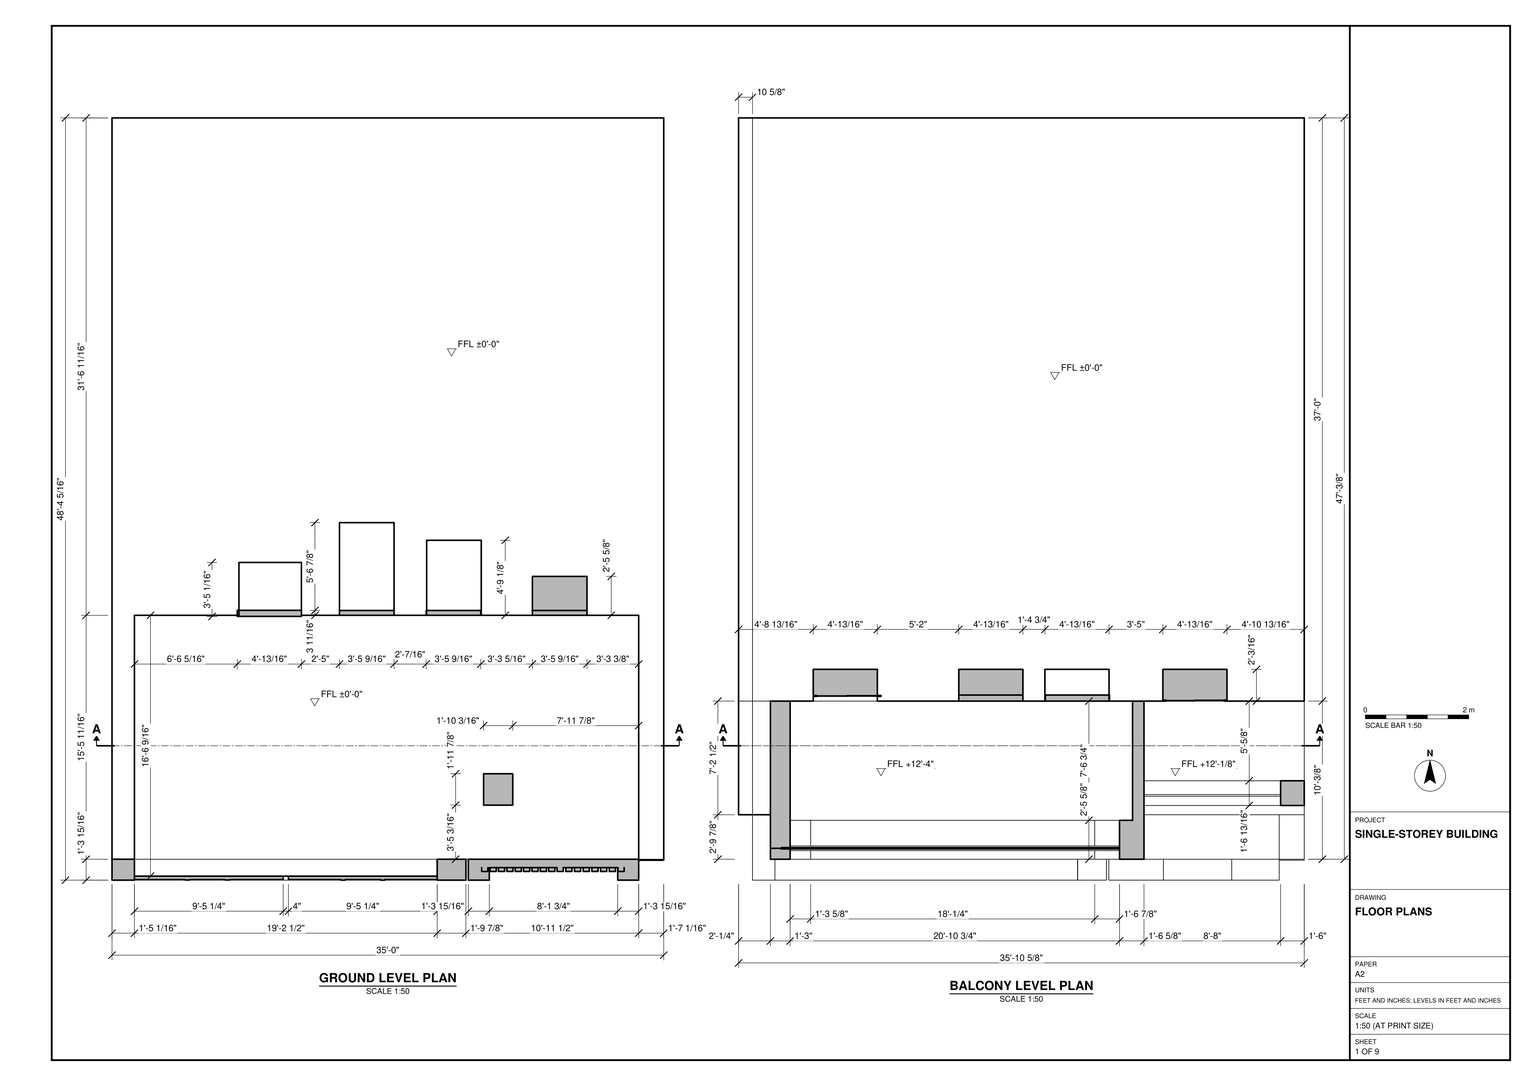
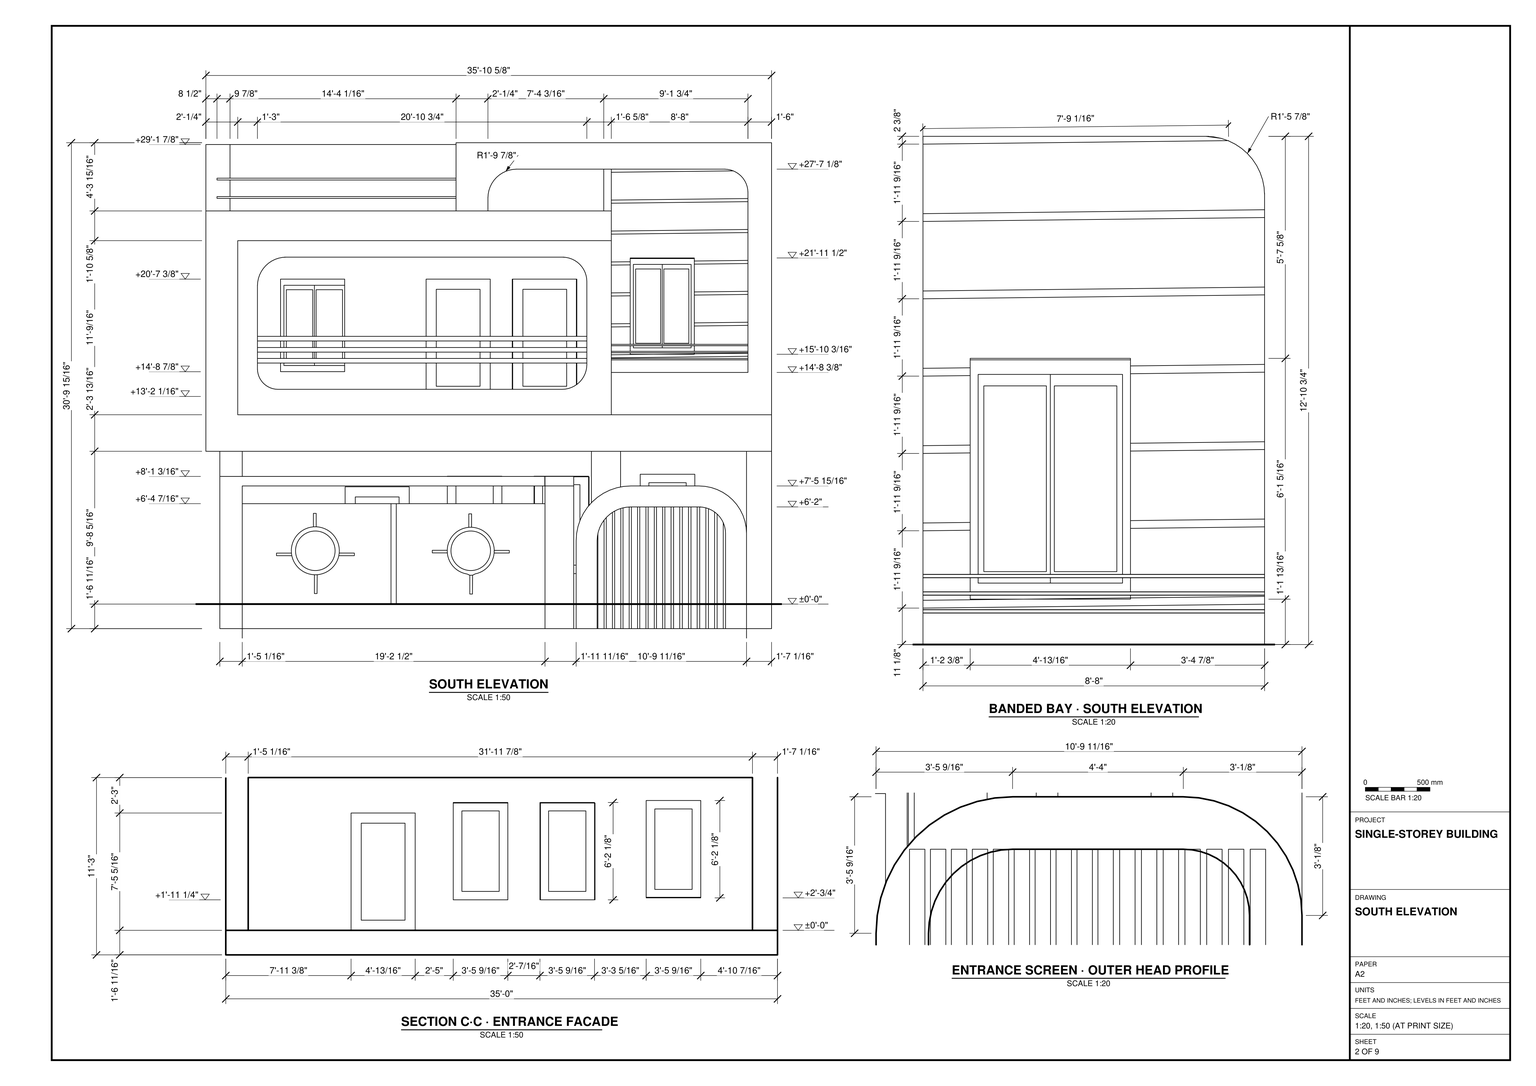
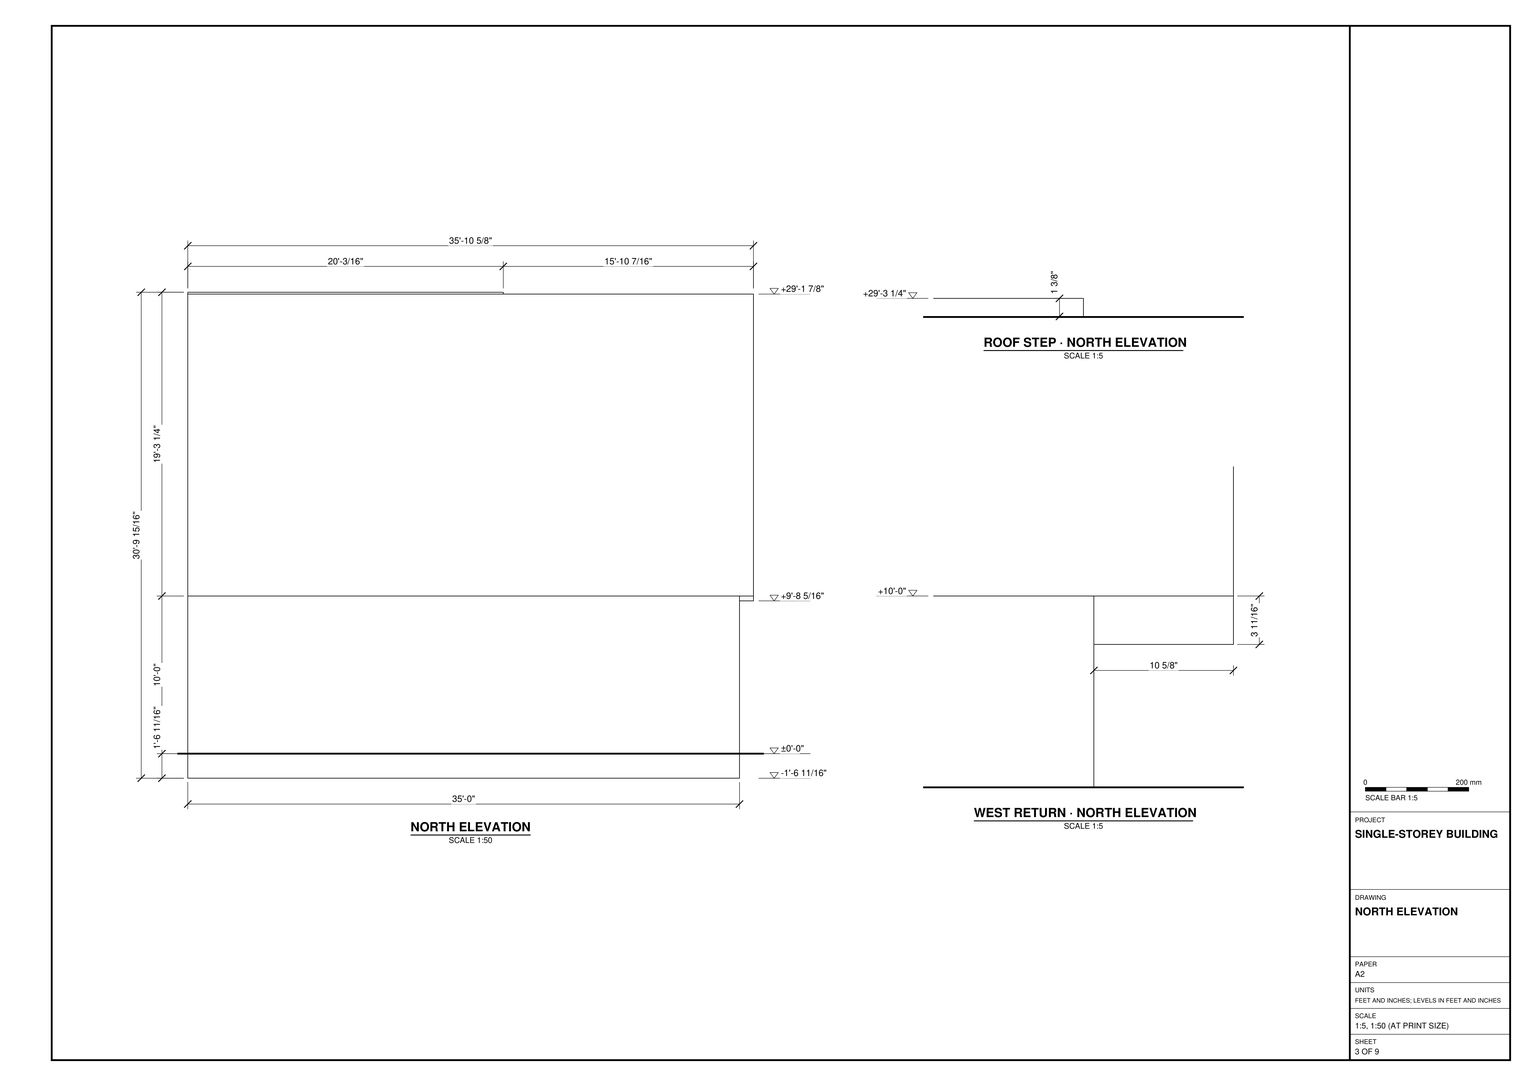
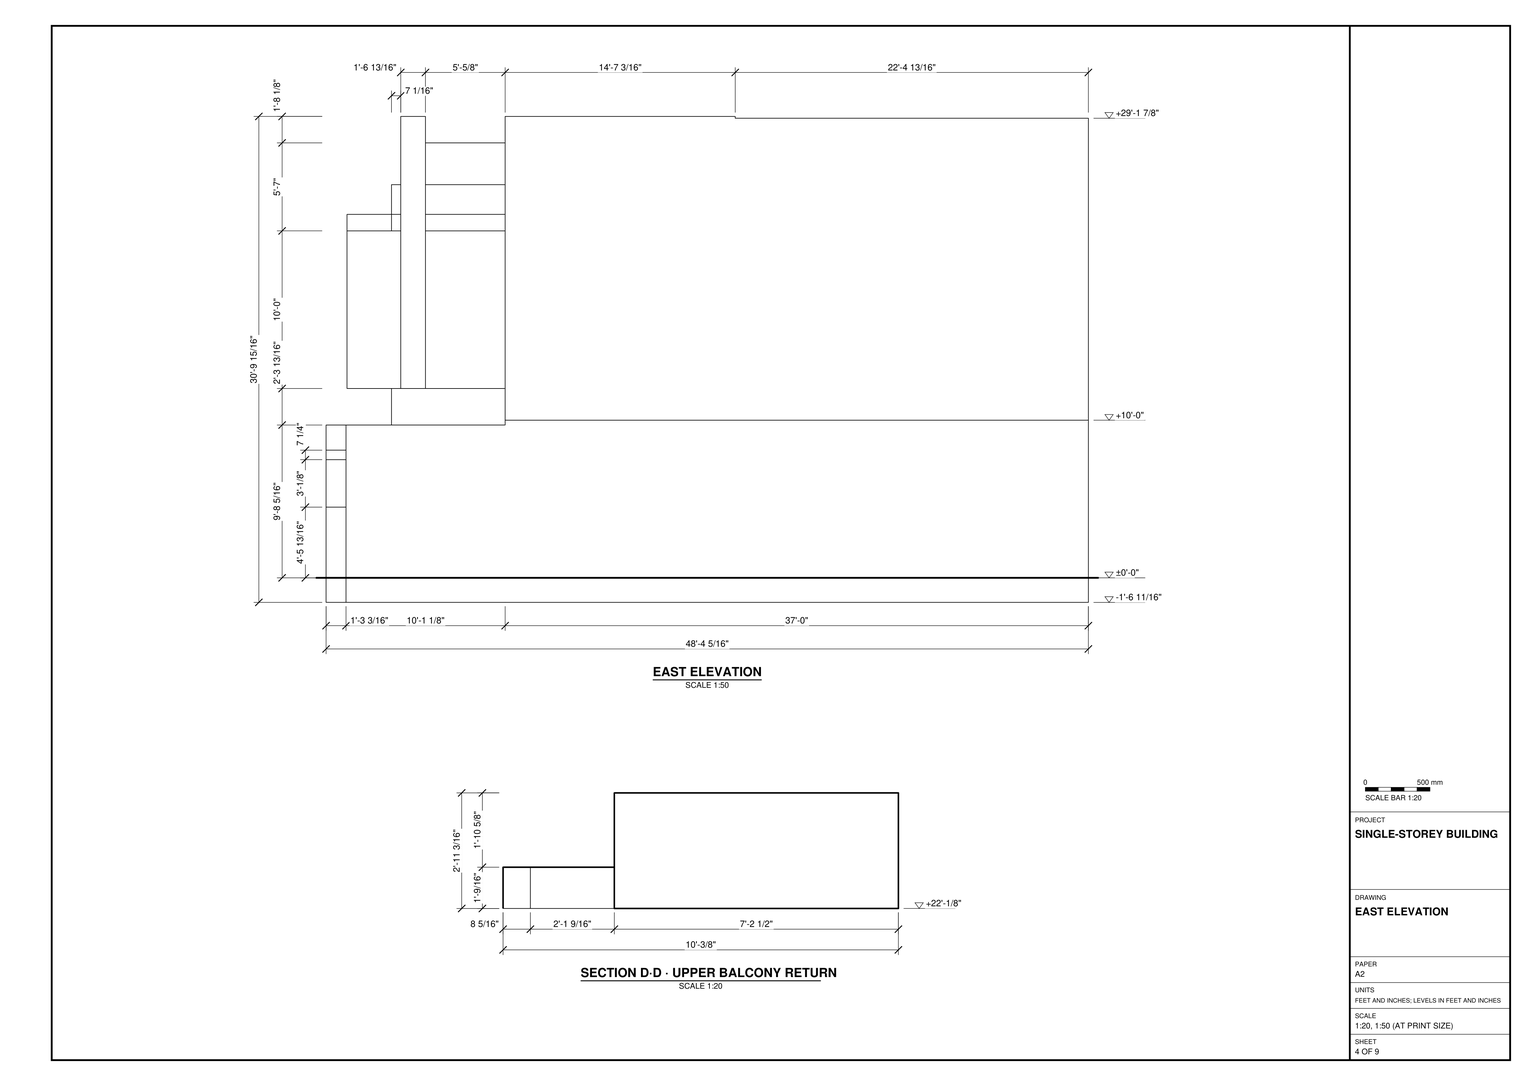
Build the house in SketchUp using the plans, elevations, sections and details in task_files/diagram_01.pdf. Work in feet and inches. Set the ground finished floor at ±0'-0". The overall model dimensions are 35'-10 5/8" wide along X, 48'-4 5/16" deep along Y and 30'-9 15/16" high along Z.

Model the base below the ground floor, the walls at their drawn thicknesses, the floor and balcony slabs, and the roof with its shallow step. At the south entrance, set the wall with the door and windows back from the gate line. Place the broad paired gate on the left and the narrower slatted screen on the right, following the curved head profile in the detail. Above the gate, form the balcony surround with rounded inner corners. Set the openings behind the horizontal guardrails. Model the adjoining banded bay with its paired window and rounded outer corner. Use the north elevation to set out the west return.

Keep walls, slabs, roof and each furniture or joinery piece shown in separate groups or components. Use components for repeated parts such as screen slats. Any decor or loose items shown may be suitable library components. Save one SketchUp model as output_files/single_storey_house_with_a_framed_south_balcony.skp.

# SketchUp Ruby script. Lengths in inches.
U = 1.inch
M = Sketchup.active_model
def pt(a) = Geom::Point3d.new(a.map { |v| v * U })
def face(e, loops, mat)
  f = e.add_face(loops[0].map { |a| pt(a) })
  loops[1..].each { |l| e.add_face(l.map { |a| pt(a) }).erase! }
  f.material = f.back_material = mat if mat
  f
end
# faces: each face lists its corners as indices into pts; further lists are holes
def faces(e, pts, list, mat = nil) = list.each { |f| face(e, (f[0].is_a?(Array) ? f : [f]).map { |l| l.map { |i| pts[i] } }, mat) }
# xy, xz, yz: faces in a plane at the given z, y or x. An outline is a flat list of corners, or four numbers for a rectangle; further outlines are holes
def ring(l) = l.size == 4 ? [[l[0], l[1]], [l[2], l[1]], [l[2], l[3]], [l[0], l[3]]] : l.each_slice(2).to_a
def flat(e, list, mat, &to3) = list.each { |f| face(e, (f[0].is_a?(Array) ? f : [f]).map { |l| ring(l).map { |u, v| to3.(u, v) } }, mat) }
def xy(e, z, list, mat = nil) = flat(e, list, mat) { |x, y| [x, y, z] }
def xz(e, y, list, mat = nil) = flat(e, list, mat) { |x, z| [x, y, z] }
def yz(e, x, list, mat = nil) = flat(e, list, mat) { |y, z| [x, y, z] }
def lines(e, pts, list) = list.each { |a, b| e.add_line(pt(pts[a]), pt(pts[b])) }
# prism: a flat outline (further loops are holes) pulled along v
def prism(e, loops, v, mat = nil)
  f = face(e, loops, mat); d = Geom::Vector3d.new(v.map { |x| x * U })
  f.pushpull(f.normal.samedirection?(d) ? d.length : -d.length)
end
def box(e, o, s, mat = nil) = prism(e, [[o, [o[0] + s[0], o[1], o[2]], [o[0] + s[0], o[1] + s[1], o[2]], [o[0], o[1] + s[1], o[2]]]], [0, 0, s[2]], mat)
def at(x, y, z, deg = 0) = Geom::Transformation.translation(pt([x, y, z])) * Geom::Transformation.rotation(ORIGIN, Z_AXIS, deg.degrees)
def axes(o, x, y, z) = Geom::Transformation.new([*x, 0, *y, 0, *z, 0, *pt(o).to_a, 1])
def part(name) = M.definitions.add(name)
# library, detail: a bought-in or finely detailed component or shape, given as its bounding box
def library(name, o, s) = part(name).tap { |d| box(d.entities, o, s) }
def detail(e, o, s) = box(e.add_group.entities, o, s)
def put(e, d, t, mat = nil) = e.add_instance(d, t).tap { |i| i.material = mat if mat }
def group(e, t, mat = nil) = e.add_group.tap { |g| g.transformation = t; g.material = mat if mat }.entities
root = M.entities
M.materials.add("Generic").color = [106, 57, 18]
M.materials.add("Generic\#1").color = [226, 203, 162]
M.materials.add("Generic\#2").color = [238, 245, 255]
M.materials.add("Generic\#3").color = [229, 166, 115]
M.materials.add("Generic\#4").color = [129, 129, 129]
M.materials.add("Generic\#5").color = [200, 187, 187]
M.materials.add("[Color M07]").color = [58, 58, 58]
M.materials.add("[Translucent Glass Gray]").color = [128, 128, 128]
M.materials["[Translucent Glass Gray]"].alpha = 0.5
M.materials.add("[Wood Veneer 01]").color = [120, 70, 37]
c1 = library("Sliding window",[0,0,0],[4.33,55.51,41.34])
c2 = part("Group\#1")
xz(c2.entities,0,[[0,0,4.6875,92.66]])
yz(c2.entities,0,[[0,0,2.9375,92.66]])
yz(c2.entities,4.6875,[[0,0,2.9375,92.66]])
c3 = part("Group\#2")
xy(c3.entities,0,[[0,0,48.8125,4.625]],"[Wood Veneer 01]")
xy(c3.entities,89.3125,[[0,0,48.8125,4.625]],"[Wood Veneer 01]")
xz(c3.entities,0,[[7.74,7.74,41.07,81.57]],"[Translucent Glass Gray]")
xz(c3.entities,0,[[[0,0,48.8125,89.3125],[7.74,7.74,41.07,81.57]]],"[Wood Veneer 01]")
xz(c3.entities,4.625,[[0,0,48.8125,89.3125]],"[Wood Veneer 01]")
yz(c3.entities,0,[[0,0,4.625,89.3125]],"[Wood Veneer 01]")
yz(c3.entities,48.8125,[[0,0,4.625,89.3125]],"[Wood Veneer 01]")
c4 = library("Group\#3",[0,0,0],[230.48,3.0625,76.4375])
xy(root,-18.6875,[[10.625,0,27.6875,15.9375],[27.6875,0,280.04,15.9375],[281.87,0,281.87,15.9375,411.5625,15.9375,411.5625,0,395.59,0,395.59,9.5625,354.12,9.5625,354.12,6.625,349.43,6.625,349.43,9.5625,297.84,9.5625,297.84,0],[280.04,2.8125,281.87,15.9375],[411.5625,15.1875,430.625,15.9375],
  [10.625,15.9375,430.625,580.3125]])
xy(root,0,[[27.6875,0,258.17,15.9375],[10.625,15.9375,27.6875,15.9375,27.6875,201.625,107.25,201.625,107.25,241.875,154.81,241.875,154.81,201.625,411.5625,201.625,411.5625,15.9375,430.625,15.9375,430.625,580.3125,10.625,580.3125],[[27.6875,15.9375,411.5625,15.9375,411.5625,201.625,154.81,201.625,154.81,241.875,107.25,241.875,107.25,201.625,27.6875,201.625],[293.5,57.12,315.6875,81.01]]])
xy(root,23.22,[[183.78,201.625,225.34,272.1875],[250.15,201.625,291.72,258.75]])
xy(root,25.16,[[330.64,201.625,372.21,231.25]])
xy(root,73.97,[[323.43,0,323.43,9.5625,349.43,9.5625,349.43,6.625,354.12,6.625,354.12,9.5625,375.42,9.5625,375.42,0]])
xy(root,86.83,[[107.25,201.625,154.81,241.875]])
xy(root,89.9375,[[27.6875,0,258,15.9375],[258.17,0,280.04,15.9375]])
xy(root,89.9375,[[323.43,0,375.42,15.9375]],"Generic\#5")
xy(root,96.91,[[183.78,201.625,225.34,272.1875],[250.15,201.625,291.72,258.75]])
xy(root,97.1875,[[10.625,0,27.6875,15.9375]])
xy(root,97.1875,[[27.6875,0,258,15.9375],[258.17,0,280.04,15.9375]],"Generic\#5")
xy(root,98.84,[[330.64,201.625,372.21,231.25]])
xy(root,116.3125,[[411.5625,15.1875,430.625,15.9375],[411.5625,15.9375,430.625,49.8125],[0,49.8125,10.625,136.3125],[10.625,49.8125,27.6875,136.3125],[27.6875,49.8125,411.5625,136.3125],
  [411.5625,49.8125,430.625,136.3125],[27.6875,136.3125,42.5625,201.625],[42.5625,136.3125,388.5,201.625],[388.5,136.3125,411.5625,201.625]])
xy(root,116.3125,[[10.625,0,27.6875,49.8125]],"Generic\#5")
xy(root,120,[[0,136.3125,10.625,580.3125],[10.625,136.3125,430.625,580.3125]])
xy(root,138.75,[[293.5,57.12,315.6875,81.01]])
xy(root,144.125,[[24.25,15.9375,39.25,24.25],[39.25,15.9375,39.25,24.25,24.25,24.25,24.25,49.8125,308.63,49.8125,308.63,15.9375],[24.25,49.8125,299.94,136.3125],[299.94,49.8125,308.63,136.3125],[308.63,49.8125,430.625,56.85],
  [308.63,75.66,430.625,136.3125]])
xy(root,148,[[24.25,24.25,39.25,136.3125],[39.25,45.5625,299.94,136.3125]])
xy(root,158.08,[[167.65,136.3125,216.46,160.5],[233.21,136.3125,282.03,160.5]])
xy(root,163.5,[[54.9,15.9375,271.13,45.5625]],"Generic\#2")
xy(root,176.35,[[308.63,56.85,412.65,75.66]],"Generic\#2")
xy(root,176.96,[[56.84,136.3125,105.65,160.5]])
xy(root,190.17,[[323,136.3125,371.82,160.5]])
xy(root,247.4,[[56.84,136.3125,105.65,160.5],[167.65,136.3125,216.46,160.5],[233.21,136.3125,282.03,160.5]])
xy(root,263.05,[[323,136.3125,371.82,160.5]])
xy(root,264.125,[[61.08,15.9375,271.46,24.25],[24.25,24.25,39.25,49.8125],[39.25,24.25,39.25,136.3125,299.94,136.3125,299.94,49.8125,290.01,49.8125,290.01,45.5625,271.46,45.5625,271.46,24.25],[271.46,24.25,290.01,45.5625],[290.01,24.25,299.94,45.5625],
  [290.01,45.5625,299.94,49.8125],[24.25,49.8125,39.25,115.875],[299.94,49.8125,308.63,115.875],[0,115.875,24.25,136.3125],[24.25,115.875,39.25,136.3125],
  [299.94,115.875,308.63,136.3125]])
xy(root,276.6875,[[299.94,15.9375,308.63,49.8125]])
xy(root,276.6875,[[24.25,15.9375,299.94,24.25],[24.25,24.25,299.94,49.8125]],"Generic\#5")
xy(root,299.3125,[[0,49.8125,302.88,49.8125,302.88,136.3125,214.71,136.3125,214.71,56.85,190.44,56.85,190.44,75.66,214.71,75.66,214.71,136.3125,0,136.3125],[302.88,49.8125,308.63,56.85],[302.88,56.85,308.63,136.3125],[18.375,136.3125,190.44,136.3125,190.44,311.47,411.1875,311.47,411.1875,565.5,18.375,565.5]])
xy(root,308.86,[[8.47,68.31,8.47,145.9,10.35,145.9,10.35,70.18,190.44,70.18,190.44,68.31]])
xy(root,310.23,[[8.47,68.31,190.44,68.31,190.44,70.18,10.35,70.18,10.35,145.9,8.47,145.9]],"Generic\#4")
xy(root,322.86,[[8.47,68.31,8.47,145.9,10.35,145.9,10.35,70.18,190.44,70.18,190.44,68.31]])
xy(root,324.23,[[8.47,68.31,190.44,68.31,190.44,70.18,10.35,70.18,10.35,145.9,8.47,145.9]],"Generic\#4")
xy(root,331.11,[[302.88,56.85,308.63,75.66],[302.88,75.66,308.63,136.3125]])
xy(root,331.11,[[236.58,56.85,302.88,75.66],[308.63,56.85,394.79,75.66]],"Generic\#2")
xy(root,349.875,[[0,136.3125,18.375,136.3125,18.375,565.5,411.1875,565.5,411.1875,311.47,430.625,311.47,430.625,580.3125,0,580.3125]],"Generic\#5")
xy(root,351.25,[[190.44,136.3125,430.625,311.47]])
xy(root,351.25,[[190.44,56.85,430.625,75.66]],"Generic\#5")
xz(root,0,[[10.625,-18.6875,27.6875,-18.6875,27.6875,89.9375,258,89.9375,258,97.1875,10.625,97.1875],[27.6875,-18.6875,258.17,0],[258.17,-18.6875,280.04,89.9375],[281.87,-18.6875,297.84,-18.6875,297.84,48.375,298.06,51.71,298.71,55,299.79,58.17,301.27,61.17,303.13,63.96,305.34,66.47,307.85,68.68,310.64,70.54,313.64,72.02,316.81,73.1,320.09,73.75,323.43,73.97,375.42,73.97,378.06,73.8,380.64,73.28,383.14,72.43,385.51,71.27,387.7,69.8,389.6875,68.0625,391.43,66.08,392.89,63.88,394.06,61.52,394.91,59.02,395.42,56.43,395.59,53.8,395.59,-18.6875,411.5625,-18.6875,411.5625,53.8,411.25,58.52,410.33,63.15,408.8125,67.63,406.72,71.87,404.09,75.8,400.98,79.35,397.42,82.47,393.49,85.1,389.25,87.1875,384.78,88.71,380.14,89.63,375.42,89.9375,323.43,89.9375,318.01,89.58,312.68,88.52,307.53,86.77,302.65,84.37,298.13,81.35,294.04,77.76,290.46,73.68,287.4375,69.16,285.03,64.28,283.29,59.13,282.23,53.8,281.87,48.375],[258.17,89.9375,280.04,97.1875],
  [10.625,97.1875,27.6875,116.3125]],"Generic\#5")
xz(root,9.5625,[[297.84,-18.6875,349.43,-18.6875,349.43,73.97,323.43,73.97,320.09,73.75,316.81,73.1,313.64,72.02,310.64,70.54,307.85,68.68,305.34,66.47,303.13,63.96,301.27,61.17,299.79,58.17,298.71,55,298.06,51.71,297.84,48.375],[354.12,-18.6875,395.59,-18.6875,395.59,53.8,395.42,56.43,394.91,59.02,394.06,61.52,392.89,63.88,391.43,66.08,389.6875,68.0625,387.7,69.8,385.51,71.27,383.14,72.43,380.64,73.28,378.06,73.8,375.42,73.97,354.12,73.97]])
xz(root,15.1875,[[411.5625,-18.6875,430.625,116.3125]],"Generic\#5")
xz(root,15.9375,[[10.625,-18.6875,27.6875,0],[27.6875,-18.6875,280.04,0],[280.04,-18.6875,281.87,0],[281.87,-18.6875,411.5625,0],[10.625,0,27.6875,97.1875],
  [258.17,0,280.04,89.9375],[281.87,0,281.87,48.375,282.23,53.8,283.29,59.13,285.03,64.28,287.4375,69.16,290.46,73.68,294.04,77.76,298.13,81.35,302.65,84.37,307.53,86.77,312.68,88.52,318.01,89.58,323.43,89.9375,375.42,89.9375,380.14,89.63,384.78,88.71,389.25,87.1875,393.49,85.1,397.42,82.47,400.98,79.35,404.09,75.8,406.72,71.87,408.8125,67.63,410.33,63.15,411.25,58.52,411.5625,53.8,411.5625,0],[27.6875,89.9375,258,97.1875],[258.17,89.9375,280.04,97.1875]])
xz(root,15.9375,[[[24.25,144.125,308.63,276.6875],[54.9,163.5,52.86,163.63,50.85,164.03,48.91,164.69,47.07,165.6,45.37,166.73,43.83,168.08,42.48,169.625,41.35,171.33,40.44,173.16,39.78,175.1,39.38,177.11,39.25,179.15,39.25,242.29,39.4375,245.14,39.99,247.94,40.91,250.65,42.18,253.21,43.76,255.58,45.65,257.73,47.79,259.61,50.17,261.2,52.73,262.46,55.43,263.38,58.23,263.9375,61.08,264.125,271.46,264.125,273.88,263.97,276.26,263.49,278.56,262.71,280.74,261.64,282.75,260.29,284.58,258.69,286.18,256.87,287.52,254.85,288.6,252.68,289.375,250.38,289.85,248,290.01,245.58,290.01,182.38,289.85,179.91,289.36,177.49,288.57,175.15,287.48,172.9375,286.11,170.89,284.48,169.03,282.62,167.4,280.57,166.03,278.35,164.9375,276.02,164.14,273.59,163.66,271.13,163.5]]],"Generic\#5")
xz(root,24.25,[[24.25,148,39.25,264.125],[39.25,242.29,39.25,264.125,61.08,264.125,58.23,263.9375,55.43,263.38,52.73,262.46,50.17,261.2,47.79,259.61,45.65,257.73,43.76,255.58,42.18,253.21,40.91,250.65,39.99,247.94,39.4375,245.14],[24.25,264.125,299.94,276.6875]])
xz(root,45.5625,[[39.25,148,39.25,179.15,39.38,177.11,39.78,175.1,40.44,173.16,41.35,171.33,42.48,169.625,43.83,168.08,45.37,166.73,47.07,165.6,48.91,164.69,50.85,164.03,52.86,163.63,54.9,163.5,271.13,163.5,273.59,163.66,276.02,164.14,278.35,164.9375,280.57,166.03,282.62,167.4,284.48,169.03,286.11,170.89,287.48,172.9375,288.57,175.15,289.36,177.49,289.85,179.91,290.01,182.38,290.01,245.58,289.85,248,289.375,250.38,288.6,252.68,287.52,254.85,286.18,256.87,284.58,258.69,282.75,260.29,280.74,261.64,278.56,262.71,276.26,263.49,273.88,263.97,271.46,264.125,299.94,264.125,299.94,148]])
xz(root,49.8125,[[299.94,264.125,308.63,276.6875]])
xz(root,49.8125,[[0,116.3125,430.625,116.3125,430.625,144.125,24.25,144.125,24.25,276.6875,308.63,276.6875,308.63,299.3125,0,299.3125]],"Generic\#1")
xz(root,56.85,[[308.63,144.125,430.625,144.125,430.625,351.25,190.44,351.25,190.44,299.3125,214.71,299.3125,214.71,309.24,214.89,312.1,215.45,314.9,216.37,317.61,217.64,320.18,219.23,322.56,221.11,324.71,223.26,326.59,225.64,328.18,228.21,329.45,230.92,330.37,233.72,330.92,236.58,331.11,394.79,331.11,397.12,330.96,399.41,330.5,401.625,329.75,403.72,328.72,405.66,327.42,407.42,325.88,408.96,324.125,410.25,322.18,411.29,320.09,412.04,317.88,412.49,315.59,412.65,313.26,412.65,176.35,308.63,176.35],[302.88,299.3125,308.63,331.11]],"Generic\#5")
xz(root,57.12,[[293.5,0,315.6875,138.75]],"Generic\#4")
xz(root,63.9,[[308.63,185.98,412.65,186.98],[308.63,191.42,412.65,192.42],[308.63,196.73,412.65,197.73]])
xz(root,65.17,[[308.63,185.93,412.65,186.93],[308.63,191.37,412.65,192.37],[308.63,196.68,412.65,197.68]])
xz(root,68.31,[[8.47,308.86,190.44,310.23],[8.47,322.86,190.44,324.23]],"Generic\#4")
xz(root,70.18,[[10.35,308.86,190.44,310.23],[10.35,322.86,190.44,324.23]])
xz(root,75.66,[[308.63,144.125,308.63,176.35,412.65,176.35,412.65,331.11,214.71,331.11,214.71,299.3125,190.44,299.3125,190.44,351.25,430.625,351.25,430.625,299.3125,413.96,299.3125,413.96,144.125],[413.96,144.125,430.625,299.3125],[214.71,309.24,214.71,331.11,236.58,331.11,233.72,330.92,230.92,330.37,228.21,329.45,225.64,328.18,223.26,326.59,221.11,324.71,219.23,322.56,217.64,320.18,216.37,317.61,215.45,314.9,214.89,312.1],[412.65,313.26,412.49,315.59,412.04,317.88,411.29,320.09,410.25,322.18,408.96,324.125,407.42,325.88,405.66,327.42,403.72,328.72,401.625,329.75,399.41,330.5,397.12,330.96,394.79,331.11,412.65,331.11]])
xz(root,81.01,[[293.5,0,315.6875,138.75]])
xz(root,136.3125,[[0,116.3125,10.625,120],[10.625,116.3125,42.5625,120],[42.5625,116.3125,388.5,120],[388.5,116.3125,430.625,120],[24.25,144.125,299.94,148],
  [299.94,144.125,308.63,148],[24.25,148,39.25,264.125],[299.94,148,308.63,264.125],[0,264.125,308.63,299.3125],[302.88,299.3125,308.63,331.11]])
xz(root,136.3125,[[[39.25,148,299.94,264.125],[167.65,158.08,216.46,247.4],[233.21,158.08,282.03,247.4],[56.84,176.96,105.65,247.4]]],"Generic\#3")
xz(root,136.3125,[[308.63,144.125,430.625,144.125,430.625,165.3,308.63,163.9],[308.63,166.27,430.625,167.67,430.625,188.85,371.82,188.17,339.09,187.8,308.63,187.45],[308.63,189.82,339.09,190.17,323,190.17,323,211.16,308.63,210.99],[371.82,190.55,430.625,191.22,430.625,212.4,371.82,211.72],[308.63,213.37,323,213.53,323,234.71,308.63,234.54],
  [371.82,214.09,430.625,214.77,430.625,235.94,371.82,235.27],[308.63,236.92,323,237.08,323,258.26,308.63,258.09],[371.82,237.64,430.625,238.32,430.625,259.49,371.82,258.82],[308.63,260.47,323,260.63,323,263.05,371.82,263.05,371.82,261.19,430.625,261.87,430.625,283.04,308.63,281.64],[308.63,284.01,430.625,285.42,430.625,306.59,308.63,305.1875],
  [190.44,299.3125,302.88,299.3125,302.88,331.11,308.63,331.11,430.625,332.51,430.625,351.25,190.44,351.25],[308.63,307.5625,430.625,308.96,430.625,330.14,308.63,328.74]],"Generic\#4")
xz(root,136.3125,[[0,299.3125,18.375,349.875]],"Generic\#5")
xz(root,136.3125,[[308.63,163.9,430.625,165.3,430.625,167.67,308.63,166.27],[308.63,187.45,339.09,187.8,371.82,188.17,430.625,188.85,430.625,191.22,371.82,190.55,371.82,190.17,339.09,190.17,308.63,189.82],[308.63,210.99,323,211.16,323,213.53,308.63,213.37],[371.82,211.72,430.625,212.4,430.625,214.77,371.82,214.09],[308.63,234.54,323,234.71,323,237.08,308.63,236.92],
  [371.82,235.27,430.625,235.94,430.625,238.32,371.82,237.64],[308.63,258.09,323,258.26,323,260.63,308.63,260.47],[371.82,258.82,430.625,259.49,430.625,261.87,371.82,261.19],[308.63,281.64,430.625,283.04,430.625,285.42,308.63,284.01],[308.63,305.1875,430.625,306.59,430.625,308.96,308.63,307.5625],
  [308.63,328.74,430.625,330.14,430.625,332.51,308.63,331.11]],"[Color M07]")
xz(root,145.9,[[8.47,308.86,10.35,310.23],[8.47,322.86,10.35,324.23]])
xz(root,160.5,[[167.65,158.08,216.46,247.4],[233.21,158.08,282.03,247.4],[56.84,176.96,105.65,247.4],[323,190.17,371.82,263.05]])
xz(root,201.625,[[[27.6875,0,107.25,0,107.25,86.83,154.81,86.83,154.81,0,411.5625,0,411.5625,116.3125,27.6875,116.3125],[183.78,23.22,225.34,96.91],[250.15,23.22,291.72,96.91],[330.64,25.16,372.21,98.84]]],"Generic\#3")
xz(root,231.25,[[330.64,25.16,372.21,98.84]])
xz(root,241.875,[[107.25,0,154.81,86.83]])
xz(root,258.75,[[250.15,23.22,291.72,96.91]])
xz(root,272.1875,[[183.78,23.22,225.34,96.91]])
xz(root,311.47,[[190.44,299.3125,190.44,351.25,430.625,351.25,430.625,349.875,411.1875,349.875,411.1875,299.3125]])
xz(root,565.5,[[18.375,299.3125,411.1875,349.875]],"Generic\#5")
xz(root,580.3125,[[10.625,-18.6875,430.625,0],[10.625,0,430.625,120],[0,120,430.625,349.875]])
yz(root,0,[[49.8125,116.3125,136.3125,264.125],[136.3125,120,580.3125,264.125],[49.8125,264.125,136.3125,299.3125]])
yz(root,0,[[136.3125,264.125,580.3125,349.875]],"Generic\#5")
yz(root,8.47,[[68.31,308.86,145.9,310.23],[68.31,322.86,145.9,324.23]],"Generic\#4")
yz(root,10.35,[[70.18,308.86,145.9,310.23],[70.18,322.86,145.9,324.23]],"Generic\#4")
yz(root,10.625,[[0,-18.6875,15.9375,97.1875],[15.9375,-18.6875,580.3125,0],[15.9375,0,15.9375,97.1875,0,97.1875,0,116.3125,136.3125,116.3125,136.3125,120,580.3125,120,580.3125,0]])
yz(root,18.375,[[136.3125,299.3125,565.5,349.875]],"Generic\#5")
yz(root,24.25,[[49.8125,144.125,136.3125,148],[49.8125,148,136.3125,264.125]])
yz(root,24.25,[[15.9375,144.125,24.25,276.6875],[24.25,144.125,49.8125,148],[24.25,148,49.8125,264.125],[24.25,264.125,49.8125,276.6875]],"Generic\#5")
yz(root,27.6875,[[0,-18.6875,15.9375,0],[0,0,15.9375,89.9375]])
yz(root,27.6875,[[15.9375,0,201.625,0,201.625,116.3125,0,116.3125,0,97.1875,15.9375,97.1875]],"Generic\#3")
yz(root,32.51,[[24.29,183.51,23.83,183.56,23.41,183.74,23.05,184.02,22.77,184.38,22.6,184.8,22.54,185.26,22.6,185.71,22.77,186.13,23.05,186.49,23.41,186.77,23.83,186.95,24.29,187.01,24.74,186.95,25.16,186.77,25.52,186.49,25.8,186.13,25.98,185.71,26.04,185.26,25.98,184.8,25.8,184.38,25.52,184.02,25.16,183.74,24.74,183.56],[24.29,191.82,23.83,191.88,23.41,192.05,23.05,192.33,22.77,192.69,22.6,193.11,22.54,193.57,22.6,194.02,22.77,194.44,23.05,194.81,23.41,195.08,23.83,195.26,24.29,195.32,24.74,195.26,25.16,195.08,25.52,194.81,25.8,194.44,25.98,194.02,26.04,193.57,25.98,193.11,25.8,192.69,25.52,192.33,25.16,192.05,24.74,191.88],[24.29,200.32,23.83,200.38,23.41,200.55,23.05,200.83,22.77,201.19,22.6,201.61,22.54,202.07,22.6,202.52,22.77,202.94,23.05,203.31,23.41,203.58,23.83,203.76,24.29,203.82,24.74,203.76,25.16,203.58,25.52,203.31,25.8,202.94,25.98,202.52,26.04,202.07,25.98,201.61,25.8,201.19,25.52,200.83,25.16,200.55,24.74,200.38]])
yz(root,39.25,[[24.25,148,45.5625,179.15],[45.5625,148,136.3125,148,136.3125,264.125,24.25,264.125,24.25,179.15,45.5625,179.15]])
yz(root,39.25,[[15.9375,179.15,24.25,242.29]],"Generic\#2")
yz(root,56.84,[[136.3125,176.96,160.5,247.4]])
yz(root,105.65,[[136.3125,176.96,160.5,247.4]])
yz(root,107.25,[[201.625,0,241.875,86.83]])
yz(root,154.81,[[201.625,0,241.875,86.83]])
yz(root,167.65,[[136.3125,158.08,160.5,247.4]])
yz(root,183.78,[[201.625,23.22,272.1875,96.91]])
yz(root,190.44,[[136.3125,299.3125,311.47,351.25],[68.31,308.86,70.18,310.23],[68.31,322.86,70.18,324.23]])
yz(root,190.44,[[[56.85,299.3125,75.66,351.25],[68.31,322.86,70.18,324.23],[68.31,308.86,70.18,310.23]]],"Generic\#5")
yz(root,214.71,[[56.85,299.3125,75.66,309.24]],"Generic\#2")
yz(root,216.46,[[136.3125,158.08,160.5,247.4]])
yz(root,225.34,[[201.625,23.22,272.1875,96.91]])
yz(root,233.21,[[136.3125,158.08,160.5,247.4]])
yz(root,250.15,[[201.625,23.22,258.75,96.91]])
yz(root,258,[[0,89.9375,15.9375,97.1875]])
yz(root,258.17,[[0,0,15.9375,89.9375],[0,89.9375,15.9375,97.1875]])
yz(root,280.04,[[0,-18.6875,15.9375,89.9375],[0,89.9375,15.9375,97.1875]])
yz(root,281.87,[[0,-18.6875,15.9375,48.375]])
yz(root,282.03,[[136.3125,158.08,160.5,247.4]])
yz(root,290.01,[[24.29,183.51,24.74,183.56,25.16,183.74,25.52,184.02,25.8,184.38,25.98,184.8,26.04,185.26,25.98,185.71,25.8,186.13,25.52,186.49,25.16,186.77,24.74,186.95,24.29,187.01,23.83,186.95,23.41,186.77,23.05,186.49,22.77,186.13,22.6,185.71,22.54,185.26,22.6,184.8,22.77,184.38,23.05,184.02,23.41,183.74,23.83,183.56],[24.29,191.82,24.74,191.88,25.16,192.05,25.52,192.33,25.8,192.69,25.98,193.11,26.04,193.57,25.98,194.02,25.8,194.44,25.52,194.81,25.16,195.08,24.74,195.26,24.29,195.32,23.83,195.26,23.41,195.08,23.05,194.81,22.77,194.44,22.6,194.02,22.54,193.57,22.6,193.11,22.77,192.69,23.05,192.33,23.41,192.05,23.83,191.88],[24.29,200.32,24.74,200.38,25.16,200.55,25.52,200.83,25.8,201.19,25.98,201.61,26.04,202.07,25.98,202.52,25.8,202.94,25.52,203.31,25.16,203.58,24.74,203.76,24.29,203.82,23.83,203.76,23.41,203.58,23.05,203.31,22.77,202.94,22.6,202.52,22.54,202.07,22.6,201.61,22.77,201.19,23.05,200.83,23.41,200.55,23.83,200.38]])
yz(root,290.01,[[[15.9375,182.38,45.5625,245.58],[24.29,200.32,24.74,200.38,25.16,200.55,25.52,200.83,25.8,201.19,25.98,201.61,26.04,202.07,25.98,202.52,25.8,202.94,25.52,203.31,25.16,203.58,24.74,203.76,24.29,203.82,23.83,203.76,23.41,203.58,23.05,203.31,22.77,202.94,22.6,202.52,22.54,202.07,22.6,201.61,22.77,201.19,23.05,200.83,23.41,200.55,23.83,200.38],[24.29,191.82,24.74,191.88,25.16,192.05,25.52,192.33,25.8,192.69,25.98,193.11,26.04,193.57,25.98,194.02,25.8,194.44,25.52,194.81,25.16,195.08,24.74,195.26,24.29,195.32,23.83,195.26,23.41,195.08,23.05,194.81,22.77,194.44,22.6,194.02,22.54,193.57,22.6,193.11,22.77,192.69,23.05,192.33,23.41,192.05,23.83,191.88],[24.29,183.51,24.74,183.56,25.16,183.74,25.52,184.02,25.8,184.38,25.98,184.8,26.04,185.26,25.98,185.71,25.8,186.13,25.52,186.49,25.16,186.77,24.74,186.95,24.29,187.01,23.83,186.95,23.41,186.77,23.05,186.49,22.77,186.13,22.6,185.71,22.54,185.26,22.6,184.8,22.77,184.38,23.05,184.02,23.41,183.74,23.83,183.56]]],"Generic\#2")
yz(root,291.72,[[201.625,23.22,258.75,96.91]])
yz(root,293.5,[[57.12,0,81.01,138.75]],"Generic\#4")
yz(root,297.84,[[0,-18.6875,9.5625,48.375]])
yz(root,299.94,[[45.5625,148,49.8125,264.125],[24.25,264.125,49.8125,276.6875]])
yz(root,299.94,[[49.8125,148,136.3125,264.125]],"Generic\#1")
yz(root,302.88,[[56.85,299.3125,136.3125,331.11]],"Generic\#5")
yz(root,308.63,[[[15.9375,144.125,56.85,144.125,56.85,176.35,75.66,176.35,75.66,144.125,136.3125,144.125,136.3125,264.125,15.9375,264.125],[65.17,196.68,63.9,196.73,63.9,197.73,65.17,197.68],[65.17,191.37,63.9,191.42,63.9,192.42,65.17,192.37],[65.17,185.93,63.9,185.98,63.9,186.98,65.17,186.93]],[15.9375,264.125,49.8125,276.6875],[49.8125,264.125,136.3125,276.6875],[49.8125,276.6875,136.3125,299.3125],[56.85,299.3125,136.3125,331.11]],"Generic\#5")
yz(root,315.6875,[[57.12,0,81.01,138.75]],"Generic\#4")
yz(root,323,[[136.3125,190.17,160.5,263.05]])
yz(root,330.64,[[201.625,25.16,231.25,98.84]])
yz(root,371.82,[[136.3125,190.17,160.5,263.05]])
yz(root,372.21,[[201.625,25.16,231.25,98.84]])
yz(root,395.59,[[0,-18.6875,9.5625,53.8]])
yz(root,411.1875,[[311.47,299.3125,565.5,349.875]],"Generic\#5")
yz(root,411.5625,[[15.1875,-18.6875,15.9375,0],[15.1875,0,15.9375,53.8],[15.1875,53.8,15.9375,89.9375],[15.1875,89.9375,15.9375,116.3125]])
yz(root,411.5625,[[15.9375,0,201.625,116.3125]],"Generic\#3")
yz(root,411.5625,[[0,-18.6875,15.1875,53.8]],"Generic\#5")
yz(root,412.65,[[65.17,185.93,65.17,186.93,63.9,186.98,63.9,185.98],[65.17,191.37,65.17,192.37,63.9,192.42,63.9,191.42],[65.17,196.68,65.17,197.68,63.9,197.73,63.9,196.73]])
yz(root,412.65,[[[56.85,176.35,75.66,313.26],[65.17,196.68,65.17,197.68,63.9,197.73,63.9,196.73],[65.17,191.37,65.17,192.37,63.9,192.42,63.9,191.42],[65.17,185.93,65.17,186.93,63.9,186.98,63.9,185.98]]],"Generic\#2")
yz(root,430.625,[[15.1875,-18.6875,580.3125,0],[15.1875,0,580.3125,0,580.3125,120,136.3125,120,136.3125,116.3125,15.1875,116.3125],[49.8125,116.3125,136.3125,144.125],[136.3125,120,580.3125,120,580.3125,349.875,311.47,349.875,311.47,351.25,136.3125,351.25]])
yz(root,430.625,[[56.85,144.125,75.66,351.25]],"Generic\#5")
p = [[281.87,15.9375,48.375],[281.87,0,48.375],[282.23,0,53.8],[282.23,15.9375,53.8],[298.06,9.5625,51.71],[298.06,0,51.71],
  [297.84,0,48.375],[297.84,9.5625,48.375],[298.71,9.5625,55],[298.71,0,55],[283.29,0,59.13],[283.29,15.9375,59.13],
  [395.59,9.5625,53.8],[395.59,0,53.8],[395.42,0,56.43],[395.42,9.5625,56.43],[411.25,15.9375,58.52],[411.25,0,58.52],
  [411.5625,0,53.8],[411.5625,15.1875,53.8],[411.5625,15.9375,53.8],[299.79,9.5625,58.17],[299.79,0,58.17],[394.91,0,59.02],
  [394.91,9.5625,59.02],[301.27,9.5625,61.17],[301.27,0,61.17],[410.33,15.9375,63.15],[410.33,0,63.15],[394.06,0,61.52],
  [394.06,9.5625,61.52],[285.03,0,64.28],[285.03,15.9375,64.28],[303.13,9.5625,63.96],[303.13,0,63.96],[392.89,0,63.88],
  [392.89,9.5625,63.88],[408.8125,15.9375,67.63],[408.8125,0,67.63],[391.43,0,66.08],[391.43,9.5625,66.08],[305.34,9.5625,66.47],
  [305.34,0,66.47],[287.4375,0,69.16],[287.4375,15.9375,69.16],[389.6875,0,68.0625],[389.6875,9.5625,68.0625],[307.85,9.5625,68.68],
  [307.85,0,68.68],[406.72,15.9375,71.87],[406.72,0,71.87],[387.7,0,69.8],[387.7,9.5625,69.8],[310.64,9.5625,70.54],
  [310.64,0,70.54],[290.46,0,73.68],[290.46,15.9375,73.68],[385.51,0,71.27],[385.51,9.5625,71.27],[313.64,9.5625,72.02],
  [313.64,0,72.02],[383.14,0,72.43],[383.14,9.5625,72.43],[404.09,15.9375,75.8],[404.09,0,75.8],[316.81,9.5625,73.1],
  [316.81,0,73.1],[380.64,0,73.28],[380.64,9.5625,73.28],[320.09,9.5625,73.75],[320.09,0,73.75],[378.06,0,73.8],
  [378.06,9.5625,73.8],[294.04,0,77.76],[294.04,15.9375,77.76],[323.43,9.5625,73.97],[323.43,0,73.97],[375.42,0,73.97],
  [375.42,9.5625,73.97],[400.98,15.9375,79.35],[400.98,0,79.35],[298.13,0,81.35],[298.13,15.9375,81.35],[397.42,15.9375,82.47],
  [397.42,0,82.47],[302.65,0,84.37],[302.65,15.9375,84.37],[393.49,15.9375,85.1],[393.49,0,85.1],[307.53,0,86.77],
  [307.53,15.9375,86.77],[389.25,15.9375,87.1875],[389.25,0,87.1875],[312.68,0,88.52],[312.68,15.9375,88.52],[384.78,15.9375,88.71],
  [384.78,0,88.71],[318.01,0,89.58],[318.01,15.9375,89.58],[380.14,15.9375,89.63],[380.14,0,89.63],[323.43,0,89.9375],
  [323.43,15.9375,89.9375],[375.42,15.9375,89.9375],[375.42,0,89.9375],[54.9,15.9375,163.5],[54.9,45.5625,163.5],[52.86,45.5625,163.63],
  [52.86,15.9375,163.63],[273.59,15.9375,163.66],[273.59,45.5625,163.66],[271.13,45.5625,163.5],[271.13,15.9375,163.5],[50.85,45.5625,164.03],
  [50.85,15.9375,164.03],[276.02,15.9375,164.14],[276.02,45.5625,164.14],[48.91,45.5625,164.69],[48.91,15.9375,164.69],[278.35,15.9375,164.9375],
  [278.35,45.5625,164.9375],[47.07,45.5625,165.6],[47.07,15.9375,165.6],[280.57,15.9375,166.03],[280.57,45.5625,166.03],[45.37,45.5625,166.73],
  [45.37,15.9375,166.73],[282.62,15.9375,167.4],[282.62,45.5625,167.4],[43.83,45.5625,168.08],[43.83,15.9375,168.08],[284.48,15.9375,169.03],
  [284.48,45.5625,169.03],[42.48,45.5625,169.625],[42.48,15.9375,169.625],[286.11,15.9375,170.89],[286.11,45.5625,170.89],[41.35,45.5625,171.33],
  [41.35,15.9375,171.33],[287.48,15.9375,172.9375],[287.48,45.5625,172.9375],[40.44,45.5625,173.16],[40.44,15.9375,173.16],[288.57,15.9375,175.15],
  [288.57,45.5625,175.15],[39.78,45.5625,175.1],[39.78,15.9375,175.1],[39.38,45.5625,177.11],[39.38,15.9375,177.11],[289.36,15.9375,177.49],
  [289.36,45.5625,177.49],[39.25,45.5625,179.15],[39.25,24.25,179.15],[39.25,15.9375,179.15],[289.85,15.9375,179.91],[289.85,45.5625,179.91],
  [290.01,15.9375,182.38],[290.01,45.5625,182.38],[290.01,24.29,183.51],[290.01,23.83,183.56],[32.51,23.83,183.56],[32.51,24.29,183.51],
  [290.01,24.74,183.56],[32.51,24.74,183.56],[290.01,23.41,183.74],[32.51,23.41,183.74],[290.01,25.16,183.74],[32.51,25.16,183.74],
  [290.01,23.05,184.02],[32.51,23.05,184.02],[290.01,25.52,184.02],[32.51,25.52,184.02],[290.01,22.77,184.38],[32.51,22.77,184.38],
  [290.01,25.8,184.38],[32.51,25.8,184.38],[290.01,22.6,184.8],[32.51,22.6,184.8],[290.01,25.98,184.8],[32.51,25.98,184.8],
  [290.01,22.54,185.26],[32.51,22.54,185.26],[290.01,26.04,185.26],[32.51,26.04,185.26],[290.01,22.6,185.71],[32.51,22.6,185.71],
  [290.01,25.98,185.71],[32.51,25.98,185.71],[290.01,22.77,186.13],[32.51,22.77,186.13],[290.01,25.8,186.13],[32.51,25.8,186.13],
  [412.65,65.17,185.93],[412.65,63.9,185.98],[308.63,63.9,185.98],[308.63,65.17,185.93],[290.01,23.05,186.49],[32.51,23.05,186.49],
  [290.01,25.52,186.49],[32.51,25.52,186.49],[290.01,23.41,186.77],[32.51,23.41,186.77],[290.01,25.16,186.77],[32.51,25.16,186.77],
  [290.01,23.83,186.95],[32.51,23.83,186.95],[290.01,24.74,186.95],[32.51,24.74,186.95],[290.01,24.29,187.01],[32.51,24.29,187.01],
  [412.65,63.9,186.98],[412.65,65.17,186.93],[308.63,65.17,186.93],[308.63,63.9,186.98],[412.65,65.17,191.37],[412.65,63.9,191.42],
  [308.63,63.9,191.42],[308.63,65.17,191.37],[290.01,24.29,191.82],[290.01,23.83,191.88],[32.51,23.83,191.88],[32.51,24.29,191.82],
  [290.01,24.74,191.88],[32.51,24.74,191.88],[290.01,23.41,192.05],[32.51,23.41,192.05],[290.01,25.16,192.05],[32.51,25.16,192.05],
  [290.01,23.05,192.33],[32.51,23.05,192.33],[290.01,25.52,192.33],[32.51,25.52,192.33],[290.01,22.77,192.69],[32.51,22.77,192.69],
  [290.01,25.8,192.69],[32.51,25.8,192.69],[412.65,63.9,192.42],[412.65,65.17,192.37],[308.63,65.17,192.37],[308.63,63.9,192.42],
  [290.01,22.6,193.11],[32.51,22.6,193.11],[290.01,25.98,193.11],[32.51,25.98,193.11],[290.01,22.54,193.57],[32.51,22.54,193.57],
  [290.01,26.04,193.57],[32.51,26.04,193.57],[290.01,22.6,194.02],[32.51,22.6,194.02],[290.01,25.98,194.02],[32.51,25.98,194.02],
  [290.01,22.77,194.44],[32.51,22.77,194.44],[290.01,25.8,194.44],[32.51,25.8,194.44],[290.01,23.05,194.81],[32.51,23.05,194.81],
  [290.01,25.52,194.81],[32.51,25.52,194.81],[290.01,23.41,195.08],[32.51,23.41,195.08],[290.01,25.16,195.08],[32.51,25.16,195.08],
  [290.01,23.83,195.26],[32.51,23.83,195.26],[290.01,24.74,195.26],[32.51,24.74,195.26],[290.01,24.29,195.32],[32.51,24.29,195.32],
  [412.65,65.17,196.68],[412.65,63.9,196.73],[308.63,63.9,196.73],[308.63,65.17,196.68],[412.65,63.9,197.73],[412.65,65.17,197.68],
  [308.63,65.17,197.68],[308.63,63.9,197.73],[290.01,24.29,200.32],[290.01,23.83,200.38],[32.51,23.83,200.38],[32.51,24.29,200.32],
  [290.01,24.74,200.38],[32.51,24.74,200.38],[290.01,23.41,200.55],[32.51,23.41,200.55],[290.01,25.16,200.55],[32.51,25.16,200.55],
  [290.01,23.05,200.83],[32.51,23.05,200.83],[290.01,25.52,200.83],[32.51,25.52,200.83],[290.01,22.77,201.19],[32.51,22.77,201.19],
  [290.01,25.8,201.19],[32.51,25.8,201.19],[290.01,22.6,201.61],[32.51,22.6,201.61],[290.01,25.98,201.61],[32.51,25.98,201.61],
  [290.01,22.54,202.07],[32.51,22.54,202.07],[290.01,26.04,202.07],[32.51,26.04,202.07],[290.01,22.6,202.52],[32.51,22.6,202.52],
  [290.01,25.98,202.52],[32.51,25.98,202.52],[290.01,22.77,202.94],[32.51,22.77,202.94],[290.01,25.8,202.94],[32.51,25.8,202.94],
  [290.01,23.05,203.31],[32.51,23.05,203.31],[290.01,25.52,203.31],[32.51,25.52,203.31],[290.01,23.41,203.58],[32.51,23.41,203.58],
  [290.01,25.16,203.58],[32.51,25.16,203.58],[290.01,23.83,203.76],[32.51,23.83,203.76],[290.01,24.74,203.76],[32.51,24.74,203.76],
  [290.01,24.29,203.82],[32.51,24.29,203.82],[39.25,24.25,242.29],[39.4375,24.25,245.14],[39.4375,15.9375,245.14],[39.25,15.9375,242.29],
  [39.99,24.25,247.94],[39.99,15.9375,247.94],[289.85,15.9375,248],[289.85,45.5625,248],[290.01,45.5625,245.58],[290.01,15.9375,245.58],
  [40.91,24.25,250.65],[40.91,15.9375,250.65],[289.375,15.9375,250.38],[289.375,45.5625,250.38],[288.6,15.9375,252.68],[288.6,45.5625,252.68],
  [42.18,24.25,253.21],[42.18,15.9375,253.21],[287.52,15.9375,254.85],[287.52,45.5625,254.85],[43.76,24.25,255.58],[43.76,15.9375,255.58],
  [286.18,15.9375,256.87],[286.18,45.5625,256.87],[45.65,24.25,257.73],[45.65,15.9375,257.73],[284.58,15.9375,258.69],[284.58,45.5625,258.69],
  [47.79,24.25,259.61],[47.79,15.9375,259.61],[282.75,15.9375,260.29],[282.75,45.5625,260.29],[50.17,24.25,261.2],[50.17,15.9375,261.2],
  [280.74,15.9375,261.64],[280.74,45.5625,261.64],[52.73,24.25,262.46],[52.73,15.9375,262.46],[278.56,15.9375,262.71],[278.56,45.5625,262.71],
  [55.43,24.25,263.38],[55.43,15.9375,263.38],[276.26,15.9375,263.49],[276.26,45.5625,263.49],[58.23,24.25,263.9375],[58.23,15.9375,263.9375],
  [273.88,15.9375,263.97],[273.88,45.5625,263.97],[61.08,24.25,264.125],[61.08,15.9375,264.125],[271.46,15.9375,264.125],[271.46,24.25,264.125],
  [271.46,45.5625,264.125],[214.89,56.85,312.1],[214.71,56.85,309.24],[214.71,75.66,309.24],[214.89,75.66,312.1],[215.45,56.85,314.9],
  [215.45,75.66,314.9],[412.65,56.85,313.26],[412.49,56.85,315.59],[412.49,75.66,315.59],[412.65,75.66,313.26],[216.37,56.85,317.61],
  [216.37,75.66,317.61],[412.04,56.85,317.88],[412.04,75.66,317.88],[217.64,56.85,320.18],[217.64,75.66,320.18],[411.29,56.85,320.09],
  [411.29,75.66,320.09],[410.25,56.85,322.18],[410.25,75.66,322.18],[219.23,56.85,322.56],[219.23,75.66,322.56],[408.96,56.85,324.125],
  [408.96,75.66,324.125],[221.11,56.85,324.71],[221.11,75.66,324.71],[407.42,56.85,325.88],[407.42,75.66,325.88],[223.26,56.85,326.59],
  [223.26,75.66,326.59],[405.66,56.85,327.42],[405.66,75.66,327.42],[225.64,56.85,328.18],[225.64,75.66,328.18],[403.72,56.85,328.72],
  [403.72,75.66,328.72],[228.21,56.85,329.45],[228.21,75.66,329.45],[401.625,56.85,329.75],[401.625,75.66,329.75],[230.92,56.85,330.37],
  [230.92,75.66,330.37],[399.41,56.85,330.5],[399.41,75.66,330.5],[233.72,56.85,330.92],[233.72,75.66,330.92],[397.12,56.85,330.96],
  [397.12,75.66,330.96],[236.58,56.85,331.11],[236.58,75.66,331.11],[394.79,56.85,331.11],[394.79,75.66,331.11],[299.94,24.25,144.125],
  [299.94,24.25,148],[290.01,24.25,144.125],[290.01,24.25,148],[39.25,24.25,144.125],[39.25,24.25,148],[299.94,49.8125,148],
  [308.63,49.8125,148],[290.01,49.8125,144.125],[290.01,49.8125,148],[299.94,49.8125,144.125],[299.94,15.9375,148],[299.94,24.25,264.125],
  [299.94,15.9375,264.125],[430.625,75.66,299.3125],[430.625,136.3125,299.3125],[412.65,56.85,331.11],[412.65,75.66,331.11],[214.71,56.85,331.11],
  [214.71,75.66,331.11],[411.5625,136.3125,0],[411.5625,136.3125,-25.9375],[27.6875,136.3125,0],[27.6875,136.3125,-25.9375],[302.35,70.81,116.3125],
  [302.35,70.81,0],[308.63,136.3125,142.72],[430.625,136.3125,144.125],[339.09,136.3125,190.17],[371.82,136.3125,190.55],[290.01,24.29,193.63],
  [32.51,24.29,193.63],[290.01,24.29,184.57],[32.51,24.29,184.57],[290.01,24.29,202.07],[32.51,24.29,202.07],[412.65,64.29,191.94],
  [308.63,64.29,191.94],[412.65,64.29,186.44],[308.63,64.29,186.44],[412.65,64.29,197.25],[308.63,64.29,197.25],[258,0,89.9375],
  [258.17,0,89.9375],[190.44,69.15,323.66],[9.32,69.15,323.66],[9.32,145.9,323.66],[9.32,69.15,309.66],[9.32,145.9,309.66],
  [190.44,69.15,309.66]]
faces(root,p,[[0,1,2,3],[3,2,10,11],[16,17,18,19,20],[27,28,17,16],[11,10,31,32],[37,38,28,27],[32,31,43,44],[49,50,38,37],
  [44,43,55,56],[63,64,50,49],[56,55,73,74],[79,80,64,63],[74,73,81,82],[83,84,80,79],[82,81,85,86],[87,88,84,83],
  [86,85,89,90],[91,92,88,87],[90,89,93,94],[95,96,92,91],[94,93,97,98],[99,100,96,95],[98,97,101,102],[103,104,100,99]],"Generic\#5")
faces(root,p,[[4,5,6,7],[8,9,5,4],[12,13,14,15],[21,22,9,8],[15,14,23,24],[25,26,22,21],[24,23,29,30],[33,34,26,25],
  [30,29,35,36],[36,35,39,40],[41,42,34,33],[40,39,45,46],[47,48,42,41],[46,45,51,52],[53,54,48,47],[52,51,57,58],
  [59,60,54,53],[58,57,61,62],[65,66,60,59],[62,61,67,68],[69,70,66,65],[68,67,71,72],[75,76,70,69],[72,71,77,78],
  [192,193,194,195],[210,211,212,213],[214,215,216,217],[236,237,238,239],[270,271,272,273],[274,275,276,277],[332,333,334,335],[338,339,333,332],
  [340,341,339,338],[344,345,341,340],[348,349,345,344],[352,353,349,348],[356,357,353,352],[360,361,357,356],[364,365,361,360],[368,369,365,364],
  [372,373,369,368],[376,377,378,373,372],[385,386,387,388],[386,391,392,387],[391,395,396,392],[395,397,398,396],[397,401,402,398],[401,405,406,402],
  [405,409,410,406],[409,413,414,410],[413,417,418,414],[417,421,422,418],[421,425,426,422],[425,429,430,426]])
faces(root,p,[[105,106,107,108],[109,110,111,112],[108,107,113,114],[115,116,110,109],[114,113,117,118],[119,120,116,115],[118,117,121,122],[123,124,120,119],
  [122,121,125,126],[127,128,124,123],[126,125,129,130],[131,132,128,127],[130,129,133,134],[135,136,132,131],[134,133,137,138],[139,140,136,135],
  [138,137,141,142],[143,144,140,139],[142,141,145,146],[146,145,147,148],[149,150,144,143],[148,147,151,152,153],[154,155,150,149],[156,157,155,154],
  [326,327,328,329],[327,330,331,328],[330,336,337,331],[336,342,343,337],[342,346,347,343],[346,350,351,347],[350,354,355,351],[354,358,359,355],
  [358,362,363,359],[362,366,367,363],[366,370,371,367],[370,374,375,371],[379,380,381,382],[383,379,382,384],[389,383,384,390],[393,389,390,394],
  [399,393,394,400],[403,399,400,404],[407,403,404,408],[411,407,408,412],[415,411,412,416],[419,415,416,420],[423,419,420,424],[427,423,424,428]],"Generic\#2")
faces(root,p,[[158,159,160,161],[162,158,161,163],[159,164,165,160],[166,162,163,167],[164,168,169,165],[170,166,167,171],[168,172,173,169],[174,170,171,175],
  [172,176,177,173],[178,174,175,179],[176,180,181,177],[182,178,179,183],[180,184,185,181],[186,182,183,187],[184,188,189,185],[190,186,187,191],
  [188,196,197,189],[198,190,191,199],[196,200,201,197],[202,198,199,203],[200,204,205,201],[206,202,203,207],[204,208,209,205],[208,206,207,209],
  [218,219,220,221],[222,218,221,223],[219,224,225,220],[226,222,223,227],[224,228,229,225],[230,226,227,231],[228,232,233,229],[234,230,231,235],
  [232,240,241,233],[242,234,235,243],[240,244,245,241],[246,242,243,247],[244,248,249,245],[250,246,247,251],[248,252,253,249],[254,250,251,255],
  [252,256,257,253],[258,254,255,259],[256,260,261,257],[262,258,259,263],[260,264,265,261],[266,262,263,267],[264,268,269,265],[268,266,267,269],
  [278,279,280,281],[282,278,281,283],[279,284,285,280],[286,282,283,287],[284,288,289,285],[290,286,287,291],[288,292,293,289],[294,290,291,295],
  [292,296,297,293],[298,294,295,299],[296,300,301,297],[302,298,299,303],[300,304,305,301],[306,302,303,307],[304,308,309,305],[310,306,307,311],
  [308,312,313,309],[314,310,311,315],[312,316,317,313],[318,314,315,319],[316,320,321,317],[322,318,319,323],[320,324,325,321],[324,322,323,325]],"Generic\#4")
lines(root,p,[[431,432],[433,434],[435,436],[437,438],[439,440],[441,437],[432,442],[443,444],[445,446],[447,448],[449,450],[451,452],
  [453,454],[455,456],[457,458],[459,460],[461,462],[463,464],[465,466],[467,468],[469,470],[471,472],[473,474],[475,476],
  [476,477],[478,479],[480,478]])
put(root,c1,axes([56.84,140.64,176.89],[0,-0.18,0],[0.92896,0,0],[0,0,1.70557]))
put(root,c1,axes([323,137.09,190.17],[0,-0.18,0],[0.87932,0,0],[0,0,1.77379]))
put(root,c2,at(349.43,6.625,-18.6875),"Generic")
put(root,c2,at(343.05,6.625,-18.6875),"Generic")
put(root,c2,at(336.68,6.625,-18.6875),"Generic")
put(root,c2,at(330.3,6.625,-18.6875),"Generic")
put(root,c2,at(323.93,6.625,-18.6875),"Generic")
put(root,c2,at(317.55,6.625,-18.6875),"Generic")
put(root,c2,at(311.18,6.625,-18.6875),"Generic")
put(root,c2,at(304.8,6.625,-18.6875),"Generic")
put(root,c2,at(298.43,6.625,-18.6875),"Generic")
put(root,c2,at(292.05,6.625,-18.6875))
put(root,c2,at(356.05,6.625,-18.6875),"Generic")
put(root,c2,at(362.68,6.625,-18.6875),"Generic")
put(root,c2,at(369.3,6.625,-18.6875),"Generic")
put(root,c2,at(375.93,6.625,-18.6875),"Generic")
put(root,c2,at(382.55,6.625,-18.6875),"Generic")
put(root,c2,at(389.18,6.625,-18.6875),"Generic")
put(root,c2,at(395.8,6.625,-18.6875))
put(root,c3,at(167.65,136.3125,158.08))
put(root,c3,at(233.59,136.3125,158.08))
put(root,c3,at(106,200.8125,0))
put(root,c3,axes([183.78,201.625,23.22],[0.85147,0,0],[0,0.798,0],[0,0,0.82992]))
put(root,c3,axes([249.78,201.625,23.22],[0.85147,0,0],[0,0.798,0],[0,0,0.82992]))
put(root,c3,axes([330.64,201.625,24.72],[0.85147,0,0],[0,0.798,0],[0,0,0.82992]))
put(root,c4,at(27.6875,0,0))
